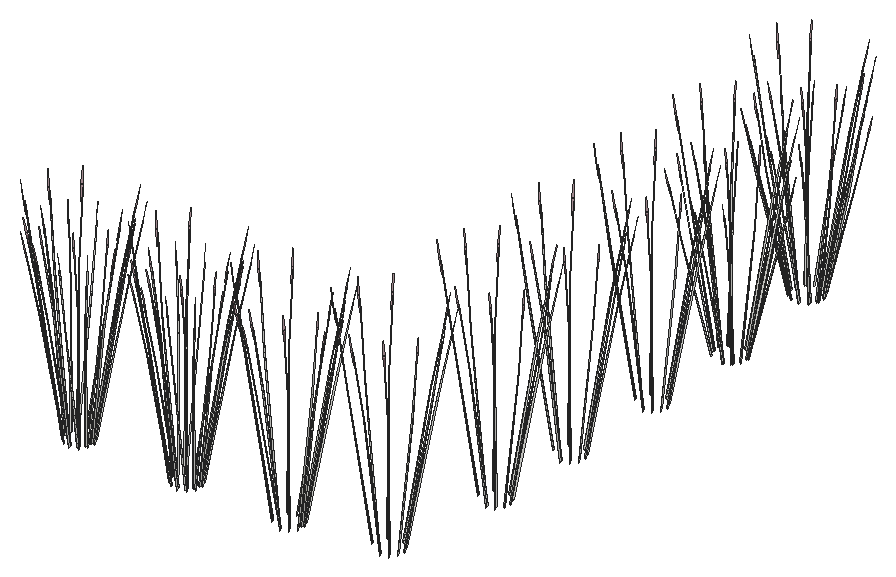
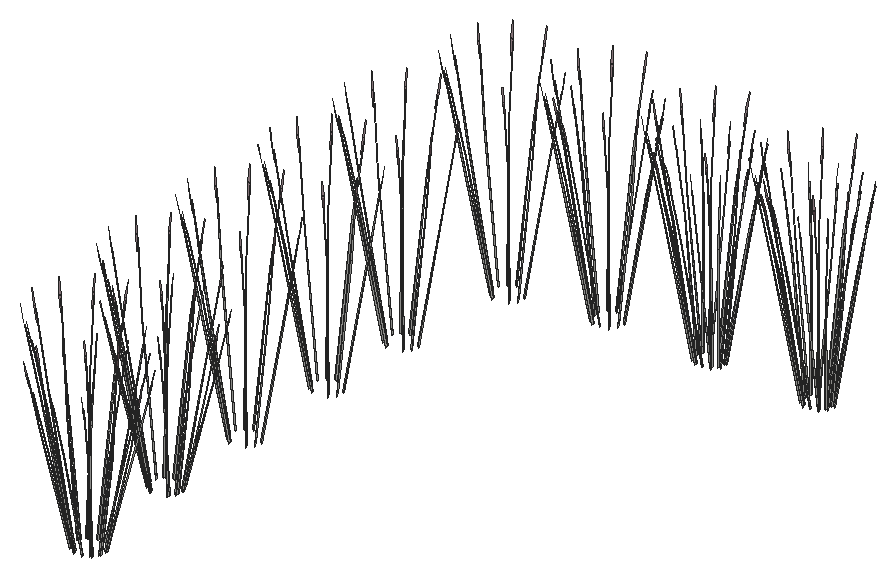
# SketchUp Ruby script. Lengths in inches.
U = 1.inch
M = Sketchup.active_model
def pt(a) = Geom::Point3d.new(a.map { |v| v * U })
def face(e, loops, mat)
  f = e.add_face(loops[0].map { |a| pt(a) })
  loops[1..].each { |l| e.add_face(l.map { |a| pt(a) }).erase! }
  f.material = f.back_material = mat if mat
  f
end
# faces: each face lists its corners as indices into pts; further lists are holes
def faces(e, pts, list, mat = nil) = list.each { |f| face(e, (f[0].is_a?(Array) ? f : [f]).map { |l| l.map { |i| pts[i] } }, mat) }
# xy, xz, yz: faces in a plane at the given z, y or x. An outline is a flat list of corners, or four numbers for a rectangle; further outlines are holes
def ring(l) = l.size == 4 ? [[l[0], l[1]], [l[2], l[1]], [l[2], l[3]], [l[0], l[3]]] : l.each_slice(2).to_a
def flat(e, list, mat, &to3) = list.each { |f| face(e, (f[0].is_a?(Array) ? f : [f]).map { |l| ring(l).map { |u, v| to3.(u, v) } }, mat) }
def xy(e, z, list, mat = nil) = flat(e, list, mat) { |x, y| [x, y, z] }
def xz(e, y, list, mat = nil) = flat(e, list, mat) { |x, z| [x, y, z] }
def yz(e, x, list, mat = nil) = flat(e, list, mat) { |y, z| [x, y, z] }
def lines(e, pts, list) = list.each { |a, b| e.add_line(pt(pts[a]), pt(pts[b])) }
# prism: a flat outline (further loops are holes) pulled along v
def prism(e, loops, v, mat = nil)
  f = face(e, loops, mat); d = Geom::Vector3d.new(v.map { |x| x * U })
  f.pushpull(f.normal.samedirection?(d) ? d.length : -d.length)
end
def box(e, o, s, mat = nil) = prism(e, [[o, [o[0] + s[0], o[1], o[2]], [o[0] + s[0], o[1] + s[1], o[2]], [o[0], o[1] + s[1], o[2]]]], [0, 0, s[2]], mat)
def at(x, y, z, deg = 0) = Geom::Transformation.translation(pt([x, y, z])) * Geom::Transformation.rotation(ORIGIN, Z_AXIS, deg.degrees)
def axes(o, x, y, z) = Geom::Transformation.new([*x, 0, *y, 0, *z, 0, *pt(o).to_a, 1])
def part(name) = M.definitions.add(name)
# library, detail: a bought-in or finely detailed component or shape, given as its bounding box
def library(name, o, s) = part(name).tap { |d| box(d.entities, o, s) }
def detail(e, o, s) = box(e.add_group.entities, o, s)
def put(e, d, t, mat = nil) = e.add_instance(d, t).tap { |i| i.material = mat if mat }
def group(e, t, mat = nil) = e.add_group.tap { |g| g.transformation = t; g.material = mat if mat }.entities
root = M.entities
M.materials.add("LightPink_Translucent").color = [144, 107, 117]
M.materials["LightPink_Translucent"].alpha = 0.75
c1 = part("blade")
p = [[2.15,0.21,22],[0,0.17,0],[0.09,0.45,0],[2.18,0.31,22],[2.29,0.31,22],[0.38,0.45,0],
  [2.48,0.24,33],[2.49,0.24,33],[2.48,0.22,33]]
faces(c1.entities,p,[[0,1,2,3],[4,5,2,3],[6,3,4,7],[8,0,3,6]])
c2 = part("seeds")
p = [[0.3,-0.1,1.38],[-0.01,-0.03,1.59],[-0.01,-0.03,0.03],[0.14,-0.07,-0.07],[0.29,-0.03,3],[0.15,0.01,3.11]]
faces(c2.entities,p,[[0,1,2,3],[1,0,4,5]],"LightPink_Translucent")
c3 = part("blade with seeds")
put(c3.entities,c1,at(0,0,0))
put(c3.entities,c2,axes([2.4,0.25,30.99],[1.5799,-0.05474,1.17369],[-0.12525,1.92788,0.29478],[-0.07173,-0.02425,1.56792]))
put(root,c3,axes([338.09,125.37,268.4],[0.18783,0.37061,0.05988],[-0.34252,0.1814,0.47138],[0.15099,-0.03579,0.71878]))
put(root,c3,axes([333.81,123.16,268.4],[0.02575,-0.41332,0.05988],[0.38885,0.01133,0.47138],[-0.14895,-0.04325,0.71878]))
put(root,c3,axes([337.34,123.02,268.4],[0.42027,0.02533,0.05988],[-0.01152,0.38243,0.47138],[0.04398,-0.14649,0.71878]))
put(root,c3,axes([337.48,126.49,268.4],[-0.02575,0.41332,0.05988],[-0.38885,-0.01133,0.47138],[0.14895,0.04325,0.71878]))
put(root,c3,axes([333.27,125.56,268.4],[-0.35109,-0.22859,0.05988],[0.2044,-0.32553,0.47138],[-0.11256,0.10524,0.71878]))
put(root,c3,axes([336.2,122.43,268.4],[0.37684,-0.18473,0.05988],[0.18445,0.33686,0.47138],[-0.03639,-0.14849,0.71878]))
put(root,c3,axes([333.21,124.29,268.4],[-0.18783,-0.37061,0.05988],[0.34252,-0.1814,0.47138],[-0.15099,0.03579,0.71878]))
put(root,c3,axes([336.39,127.17,268.4],[-0.23243,0.34529,0.05988],[-0.331,-0.20103,0.47138],[0.10701,0.1107,0.71878]))
put(root,c3,axes([333.96,126.63,268.4],[-0.42027,-0.02533,0.05988],[0.01152,-0.38243,0.47138],[-0.04398,0.14649,0.71878]))
put(root,c3,axes([332.69,140.49,268.4],[0.23243,-0.34529,0.05988],[0.331,0.20103,0.47138],[-0.10701,-0.1107,0.71878]))
put(root,c3,axes([332.89,145.23,268.4],[-0.37684,0.18473,0.05988],[-0.18445,-0.33686,0.47138],[0.03639,0.14849,0.71878]))
put(root,c3,axes([335.82,142.11,268.4],[0.35109,0.22859,0.05988],[-0.2044,0.32553,0.47138],[0.11256,-0.10524,0.71878]))
put(root,c3,axes([335.87,143.38,268.4],[0.18783,0.37061,0.05988],[-0.34252,0.1814,0.47138],[0.15099,-0.03579,0.71878]))
put(root,c3,axes([331.6,141.17,268.4],[0.02575,-0.41332,0.05988],[0.38885,0.01133,0.47138],[-0.14895,-0.04325,0.71878]))
put(root,c3,axes([335.125,141.03,268.4],[0.42027,0.02533,0.05988],[-0.01152,0.38243,0.47138],[0.04398,-0.14649,0.71878]))
put(root,c3,axes([335.27,144.5,268.4],[-0.02575,0.41332,0.05988],[-0.38885,-0.01133,0.47138],[0.14895,0.04325,0.71878]))
put(root,c3,axes([331.05,143.57,268.4],[-0.35109,-0.22859,0.05988],[0.2044,-0.32553,0.47138],[-0.11256,0.10524,0.71878]))
put(root,c3,axes([333.98,140.44,268.4],[0.37684,-0.18473,0.05988],[0.18445,0.33686,0.47138],[-0.03639,-0.14849,0.71878]))
put(root,c3,axes([331,142.3,268.4],[-0.18783,-0.37061,0.05988],[0.34252,-0.1814,0.47138],[-0.15099,0.03579,0.71878]))
put(root,c3,axes([334.18,145.18,268.4],[-0.23243,0.34529,0.05988],[-0.331,-0.20103,0.47138],[0.10701,0.1107,0.71878]))
put(root,c3,axes([331.74,144.64,268.4],[-0.42027,-0.02533,0.05988],[0.01152,-0.38243,0.47138],[-0.04398,0.14649,0.71878]))
put(root,c3,axes([285.95,54.78,268.41],[0.50393,0.1421,0.447],[-0.17232,0.46717,0.36857],[-0.03028,-0.18372,0.92496]))
put(root,c3,axes([287.41,58.67,268.41],[-0.37709,0.35815,0.447],[-0.32522,-0.38035,0.36857],[0.17692,0.06607,0.92496]))
put(root,c3,axes([287.9375,57.55,268.41],[-0.14449,0.4956,0.447],[-0.47502,-0.16947,0.36857],[0.1868,-0.02978,0.92496]))
put(root,c3,axes([283.25,57.97,268.41],[-0.12683,-0.50025,0.447],[0.49754,-0.08682,0.36857],[-0.14663,0.11765,0.92496]))
put(root,c3,axes([283.98,58.98,268.41],[-0.36417,-0.37086,0.447],[0.38674,-0.31985,0.36857],[-0.06718,0.174,0.92496]))
put(root,c3,axes([287.1,55.3,268.41],[0.36417,0.37086,0.447],[-0.38674,0.31985,0.36857],[0.06718,-0.174,0.92496]))
put(root,c3,axes([283.14,56.73,268.41],[0.14449,-0.4956,0.447],[0.47502,0.16947,0.36857],[-0.1868,0.02978,0.92496]))
put(root,c3,axes([287.82,56.3125,268.41],[0.12683,0.50025,0.447],[-0.49754,0.08682,0.36857],[0.14663,-0.11765,0.92496]))
put(root,c3,axes([286.38,59.39,268.41],[-0.50866,0.12474,0.447],[-0.08828,-0.48932,0.36857],[0.11963,0.14421,0.92496]))
put(root,c3,axes([303.17,54.78,268.41],[0.50393,0.1421,0.447],[-0.17232,0.46717,0.36857],[-0.03028,-0.18372,0.92496]))
put(root,c3,axes([304.63,58.67,268.41],[-0.37709,0.35815,0.447],[-0.32522,-0.38035,0.36857],[0.17692,0.06607,0.92496]))
put(root,c3,axes([305.16,57.55,268.41],[-0.14449,0.4956,0.447],[-0.47502,-0.16947,0.36857],[0.1868,-0.02978,0.92496]))
put(root,c3,axes([300.47,57.97,268.41],[-0.12683,-0.50025,0.447],[0.49754,-0.08682,0.36857],[-0.14663,0.11765,0.92496]))
put(root,c3,axes([301.2,58.98,268.41],[-0.36417,-0.37086,0.447],[0.38674,-0.31985,0.36857],[-0.06718,0.174,0.92496]))
put(root,c3,axes([304.32,55.3,268.41],[0.36417,0.37086,0.447],[-0.38674,0.31985,0.36857],[0.06718,-0.174,0.92496]))
put(root,c3,axes([300.36,56.73,268.41],[0.14449,-0.4956,0.447],[0.47502,0.16947,0.36857],[-0.1868,0.02978,0.92496]))
put(root,c3,axes([305.04,56.3125,268.41],[0.12683,0.50025,0.447],[-0.49754,0.08682,0.36857],[0.14663,-0.11765,0.92496]))
put(root,c3,axes([303.6,59.39,268.41],[-0.50866,0.12474,0.447],[-0.08828,-0.48932,0.36857],[0.11963,0.14421,0.92496]))
put(root,c3,axes([319.53,54.78,268.41],[0.50393,0.1421,0.447],[-0.17232,0.46717,0.36857],[-0.03028,-0.18372,0.92496]))
put(root,c3,axes([320.99,58.67,268.41],[-0.37709,0.35815,0.447],[-0.32522,-0.38035,0.36857],[0.17692,0.06607,0.92496]))
put(root,c3,axes([321.52,57.55,268.41],[-0.14449,0.4956,0.447],[-0.47502,-0.16947,0.36857],[0.1868,-0.02978,0.92496]))
put(root,c3,axes([316.84,57.97,268.41],[-0.12683,-0.50025,0.447],[0.49754,-0.08682,0.36857],[-0.14663,0.11765,0.92496]))
put(root,c3,axes([317.5625,58.98,268.41],[-0.36417,-0.37086,0.447],[0.38674,-0.31985,0.36857],[-0.06718,0.174,0.92496]))
put(root,c3,axes([320.68,55.3,268.41],[0.36417,0.37086,0.447],[-0.38674,0.31985,0.36857],[0.06718,-0.174,0.92496]))
put(root,c3,axes([316.72,56.73,268.41],[0.14449,-0.4956,0.447],[0.47502,0.16947,0.36857],[-0.1868,0.02978,0.92496]))
put(root,c3,axes([321.41,56.3125,268.41],[0.12683,0.50025,0.447],[-0.49754,0.08682,0.36857],[0.14663,-0.11765,0.92496]))
put(root,c3,axes([319.96,59.39,268.41],[-0.50866,0.12474,0.447],[-0.08828,-0.48932,0.36857],[0.11963,0.14421,0.92496]))
put(root,c3,axes([333.37,57.48,268.41],[0.50393,0.1421,0.447],[-0.17232,0.46717,0.36857],[-0.03028,-0.18372,0.92496]))
put(root,c3,axes([334.82,61.37,268.41],[-0.37709,0.35815,0.447],[-0.32522,-0.38035,0.36857],[0.17692,0.06607,0.92496]))
put(root,c3,axes([335.35,60.24,268.41],[-0.14449,0.4956,0.447],[-0.47502,-0.16947,0.36857],[0.1868,-0.02978,0.92496]))
put(root,c3,axes([330.67,60.66,268.41],[-0.12683,-0.50025,0.447],[0.49754,-0.08682,0.36857],[-0.14663,0.11765,0.92496]))
put(root,c3,axes([331.4,61.67,268.41],[-0.36417,-0.37086,0.447],[0.38674,-0.31985,0.36857],[-0.06718,0.174,0.92496]))
put(root,c3,axes([334.51,58,268.41],[0.36417,0.37086,0.447],[-0.38674,0.31985,0.36857],[0.06718,-0.174,0.92496]))
put(root,c3,axes([330.55,59.43,268.41],[0.14449,-0.4956,0.447],[0.47502,0.16947,0.36857],[-0.1868,0.02978,0.92496]))
put(root,c3,axes([335.24,59.01,268.41],[0.12683,0.50025,0.447],[-0.49754,0.08682,0.36857],[0.14663,-0.11765,0.92496]))
put(root,c3,axes([333.79,62.08,268.41],[-0.50866,0.12474,0.447],[-0.08828,-0.48932,0.36857],[0.11963,0.14421,0.92496]))
put(root,c3,axes([336.0625,75.32,268.41],[0.50393,0.1421,0.447],[-0.17232,0.46717,0.36857],[-0.03028,-0.18372,0.92496]))
put(root,c3,axes([337.52,79.22,268.41],[-0.37709,0.35815,0.447],[-0.32522,-0.38035,0.36857],[0.17692,0.06607,0.92496]))
put(root,c3,axes([338.05,78.09,268.41],[-0.14449,0.4956,0.447],[-0.47502,-0.16947,0.36857],[0.1868,-0.02978,0.92496]))
put(root,c3,axes([333.37,78.51,268.41],[-0.12683,-0.50025,0.447],[0.49754,-0.08682,0.36857],[-0.14663,0.11765,0.92496]))
put(root,c3,axes([334.09,79.52,268.41],[-0.36417,-0.37086,0.447],[0.38674,-0.31985,0.36857],[-0.06718,0.174,0.92496]))
put(root,c3,axes([337.21,75.84,268.41],[0.36417,0.37086,0.447],[-0.38674,0.31985,0.36857],[0.06718,-0.174,0.92496]))
put(root,c3,axes([333.25,77.28,268.41],[0.14449,-0.4956,0.447],[0.47502,0.16947,0.36857],[-0.1868,0.02978,0.92496]))
put(root,c3,axes([337.93,76.86,268.41],[0.12683,0.50025,0.447],[-0.49754,0.08682,0.36857],[0.14663,-0.11765,0.92496]))
put(root,c3,axes([336.49,79.93,268.41],[-0.50866,0.12474,0.447],[-0.08828,-0.48932,0.36857],[0.11963,0.14421,0.92496]))
put(root,c3,axes([336.0625,90.21,268.41],[0.50393,0.1421,0.447],[-0.17232,0.46717,0.36857],[-0.03028,-0.18372,0.92496]))
put(root,c3,axes([337.52,94.1,268.41],[-0.37709,0.35815,0.447],[-0.32522,-0.38035,0.36857],[0.17692,0.06607,0.92496]))
put(root,c3,axes([338.05,92.98,268.41],[-0.14449,0.4956,0.447],[-0.47502,-0.16947,0.36857],[0.1868,-0.02978,0.92496]))
put(root,c3,axes([333.37,93.4,268.41],[-0.12683,-0.50025,0.447],[0.49754,-0.08682,0.36857],[-0.14663,0.11765,0.92496]))
put(root,c3,axes([334.09,94.41,268.41],[-0.36417,-0.37086,0.447],[0.38674,-0.31985,0.36857],[-0.06718,0.174,0.92496]))
put(root,c3,axes([337.21,90.73,268.41],[0.36417,0.37086,0.447],[-0.38674,0.31985,0.36857],[0.06718,-0.174,0.92496]))
put(root,c3,axes([333.25,92.16,268.41],[0.14449,-0.4956,0.447],[0.47502,0.16947,0.36857],[-0.1868,0.02978,0.92496]))
put(root,c3,axes([337.93,91.74,268.41],[0.12683,0.50025,0.447],[-0.49754,0.08682,0.36857],[0.14663,-0.11765,0.92496]))
put(root,c3,axes([336.49,94.82,268.41],[-0.50866,0.12474,0.447],[-0.08828,-0.48932,0.36857],[0.11963,0.14421,0.92496]))
put(root,c3,axes([336.0625,106.63,268.41],[0.50393,0.1421,0.447],[-0.17232,0.46717,0.36857],[-0.03028,-0.18372,0.92496]))
put(root,c3,axes([337.52,110.52,268.41],[-0.37709,0.35815,0.447],[-0.32522,-0.38035,0.36857],[0.17692,0.06607,0.92496]))
put(root,c3,axes([338.05,109.4,268.41],[-0.14449,0.4956,0.447],[-0.47502,-0.16947,0.36857],[0.1868,-0.02978,0.92496]))
put(root,c3,axes([333.37,109.82,268.41],[-0.12683,-0.50025,0.447],[0.49754,-0.08682,0.36857],[-0.14663,0.11765,0.92496]))
put(root,c3,axes([334.09,110.83,268.41],[-0.36417,-0.37086,0.447],[0.38674,-0.31985,0.36857],[-0.06718,0.174,0.92496]))
put(root,c3,axes([337.21,107.15,268.41],[0.36417,0.37086,0.447],[-0.38674,0.31985,0.36857],[0.06718,-0.174,0.92496]))
put(root,c3,axes([333.25,108.58,268.41],[0.14449,-0.4956,0.447],[0.47502,0.16947,0.36857],[-0.1868,0.02978,0.92496]))
put(root,c3,axes([337.93,108.16,268.41],[0.12683,0.50025,0.447],[-0.49754,0.08682,0.36857],[0.14663,-0.11765,0.92496]))
put(root,c3,axes([336.49,111.24,268.41],[-0.50866,0.12474,0.447],[-0.08828,-0.48932,0.36857],[0.11963,0.14421,0.92496]))
put(root,c3,axes([336.0625,122.47,268.41],[0.50393,0.1421,0.447],[-0.17232,0.46717,0.36857],[-0.03028,-0.18372,0.92496]))
put(root,c3,axes([337.52,126.36,268.41],[-0.37709,0.35815,0.447],[-0.32522,-0.38035,0.36857],[0.17692,0.06607,0.92496]))
put(root,c3,axes([338.05,125.24,268.41],[-0.14449,0.4956,0.447],[-0.47502,-0.16947,0.36857],[0.1868,-0.02978,0.92496]))
put(root,c3,axes([333.37,125.66,268.41],[-0.12683,-0.50025,0.447],[0.49754,-0.08682,0.36857],[-0.14663,0.11765,0.92496]))
put(root,c3,axes([334.09,126.67,268.41],[-0.36417,-0.37086,0.447],[0.38674,-0.31985,0.36857],[-0.06718,0.174,0.92496]))
put(root,c3,axes([337.21,122.99,268.41],[0.36417,0.37086,0.447],[-0.38674,0.31985,0.36857],[0.06718,-0.174,0.92496]))
put(root,c3,axes([333.25,124.42,268.41],[0.14449,-0.4956,0.447],[0.47502,0.16947,0.36857],[-0.1868,0.02978,0.92496]))
put(root,c3,axes([337.93,124,268.41],[0.12683,0.50025,0.447],[-0.49754,0.08682,0.36857],[0.14663,-0.11765,0.92496]))
put(root,c3,axes([336.49,127.08,268.41],[-0.50866,0.12474,0.447],[-0.08828,-0.48932,0.36857],[0.11963,0.14421,0.92496]))
put(root,c3,axes([333.85,140.48,268.41],[0.50393,0.1421,0.447],[-0.17232,0.46717,0.36857],[-0.03028,-0.18372,0.92496]))
put(root,c3,axes([335.31,144.37,268.41],[-0.37709,0.35815,0.447],[-0.32522,-0.38035,0.36857],[0.17692,0.06607,0.92496]))
put(root,c3,axes([335.83,143.25,268.41],[-0.14449,0.4956,0.447],[-0.47502,-0.16947,0.36857],[0.1868,-0.02978,0.92496]))
put(root,c3,axes([331.15,143.67,268.41],[-0.12683,-0.50025,0.447],[0.49754,-0.08682,0.36857],[-0.14663,0.11765,0.92496]))
put(root,c3,axes([331.875,144.68,268.41],[-0.36417,-0.37086,0.447],[0.38674,-0.31985,0.36857],[-0.06718,0.174,0.92496]))
put(root,c3,axes([334.99,141,268.41],[0.36417,0.37086,0.447],[-0.38674,0.31985,0.36857],[0.06718,-0.174,0.92496]))
put(root,c3,axes([331.04,142.43,268.41],[0.14449,-0.4956,0.447],[0.47502,0.16947,0.36857],[-0.1868,0.02978,0.92496]))
put(root,c3,axes([335.72,142.01,268.41],[0.12683,0.50025,0.447],[-0.49754,0.08682,0.36857],[0.14663,-0.11765,0.92496]))
put(root,c3,axes([334.28,145.09,268.41],[-0.50866,0.12474,0.447],[-0.08828,-0.48932,0.36857],[0.11963,0.14421,0.92496]))
put(root,c3,axes([285.13,59.15,268.7],[0.15418,-0.41799,0.32977],[0.44981,0.12192,-0.42575],[0.04124,0.16829,0.81462]))
put(root,c3,axes([285.95,55.12,268.7],[-0.15418,0.41799,0.32977],[-0.44981,-0.12192,-0.42575],[-0.04124,-0.16829,0.81462]))
put(root,c3,axes([287.11,58.49,268.7],[-0.29098,-0.34031,0.32977],[0.33226,-0.32215,-0.42575],[0.16881,0.04902,0.81462]))
put(root,c3,axes([287.59,57.54,268.7],[-0.42502,-0.15163,0.32977],[0.12396,-0.44238,-0.42575],[0.17112,-0.04056,0.81462]))
put(root,c3,axes([283.97,55.78,268.7],[0.29098,0.34031,0.32977],[-0.33226,0.32215,-0.42575],[-0.16881,-0.04902,0.81462]))
put(root,c3,axes([284.16,58.68,268.7],[0.34603,-0.28618,0.32977],[0.32756,0.32677,-0.42575],[-0.04984,0.16603,0.81462]))
put(root,c3,axes([283.56,57.8,268.7],[0.44516,-0.07768,0.32977],[0.11755,0.44407,-0.42575],[-0.12757,0.11927,0.81462]))
put(root,c3,axes([286.21,59.08,268.7],[-0.07899,-0.43781,0.32977],[0.45153,-0.11561,-0.42575],[0.12128,0.12546,0.81462]))
put(root,c3,axes([287.52,56.48,268.7],[-0.44516,0.07768,0.32977],[-0.11755,-0.44407,-0.42575],[0.12757,-0.11927,0.81462]))
put(root,c3,axes([283.49,56.74,268.7],[0.42502,0.15163,0.32977],[-0.12396,0.44238,-0.42575],[-0.17112,0.04056,0.81462]))
put(root,c3,axes([286.92,55.59,268.7],[-0.34603,0.28618,0.32977],[-0.32756,-0.32677,-0.42575],[0.04984,-0.16603,0.81462]))
put(root,c3,axes([284.87,55.19,268.7],[0.07899,0.43781,0.32977],[-0.45153,0.11561,-0.42575],[-0.12128,-0.12546,0.81462]))
put(root,c3,axes([302.35,59.15,268.7],[0.15418,-0.41799,0.32977],[0.44981,0.12192,-0.42575],[0.04124,0.16829,0.81462]))
put(root,c3,axes([303.17,55.12,268.7],[-0.15418,0.41799,0.32977],[-0.44981,-0.12192,-0.42575],[-0.04124,-0.16829,0.81462]))
put(root,c3,axes([304.33,58.49,268.7],[-0.29098,-0.34031,0.32977],[0.33226,-0.32215,-0.42575],[0.16881,0.04902,0.81462]))
put(root,c3,axes([304.81,57.54,268.7],[-0.42502,-0.15163,0.32977],[0.12396,-0.44238,-0.42575],[0.17112,-0.04056,0.81462]))
put(root,c3,axes([301.1875,55.78,268.7],[0.29098,0.34031,0.32977],[-0.33226,0.32215,-0.42575],[-0.16881,-0.04902,0.81462]))
put(root,c3,axes([301.38,58.68,268.7],[0.34603,-0.28618,0.32977],[0.32756,0.32677,-0.42575],[-0.04984,0.16603,0.81462]))
put(root,c3,axes([300.78,57.8,268.7],[0.44516,-0.07768,0.32977],[0.11755,0.44407,-0.42575],[-0.12757,0.11927,0.81462]))
put(root,c3,axes([303.43,59.08,268.7],[-0.07899,-0.43781,0.32977],[0.45153,-0.11561,-0.42575],[0.12128,0.12546,0.81462]))
put(root,c3,axes([304.74,56.48,268.7],[-0.44516,0.07768,0.32977],[-0.11755,-0.44407,-0.42575],[0.12757,-0.11927,0.81462]))
put(root,c3,axes([300.71,56.74,268.7],[0.42502,0.15163,0.32977],[-0.12396,0.44238,-0.42575],[-0.17112,0.04056,0.81462]))
put(root,c3,axes([304.14,55.59,268.7],[-0.34603,0.28618,0.32977],[-0.32756,-0.32677,-0.42575],[0.04984,-0.16603,0.81462]))
put(root,c3,axes([302.09,55.19,268.7],[0.07899,0.43781,0.32977],[-0.45153,0.11561,-0.42575],[-0.12128,-0.12546,0.81462]))
put(root,c3,axes([318.71,59.15,268.7],[0.15418,-0.41799,0.32977],[0.44981,0.12192,-0.42575],[0.04124,0.16829,0.81462]))
put(root,c3,axes([319.53,55.12,268.7],[-0.15418,0.41799,0.32977],[-0.44981,-0.12192,-0.42575],[-0.04124,-0.16829,0.81462]))
put(root,c3,axes([320.69,58.49,268.7],[-0.29098,-0.34031,0.32977],[0.33226,-0.32215,-0.42575],[0.16881,0.04902,0.81462]))
put(root,c3,axes([321.17,57.54,268.7],[-0.42502,-0.15163,0.32977],[0.12396,-0.44238,-0.42575],[0.17112,-0.04056,0.81462]))
put(root,c3,axes([317.55,55.78,268.7],[0.29098,0.34031,0.32977],[-0.33226,0.32215,-0.42575],[-0.16881,-0.04902,0.81462]))
